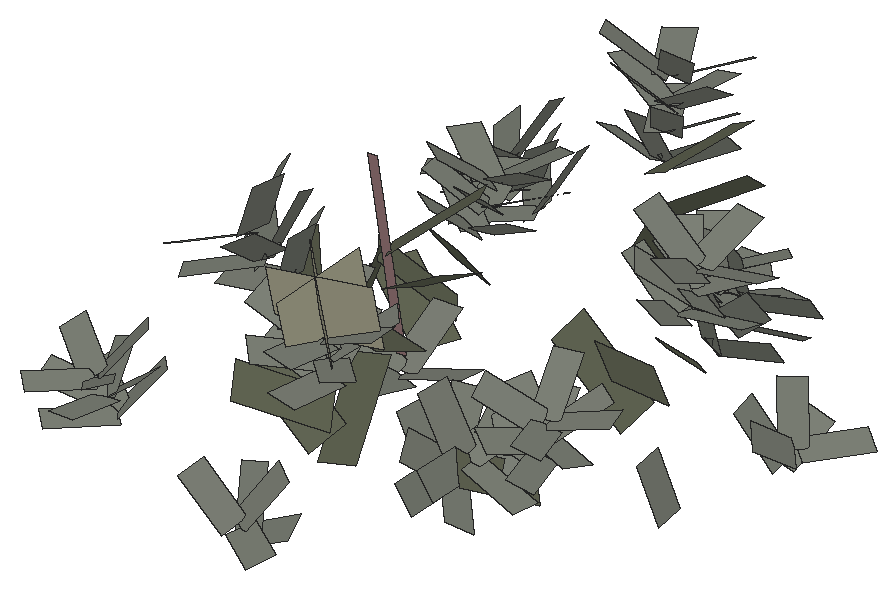
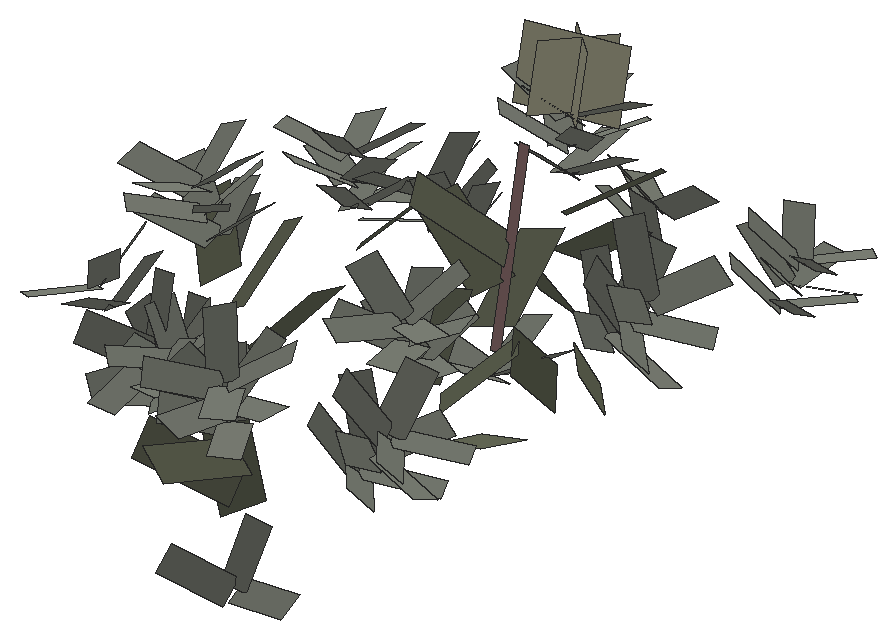
# SketchUp Ruby script. Lengths in inches.
U = 1.inch
M = Sketchup.active_model
def pt(a) = Geom::Point3d.new(a.map { |v| v * U })
def face(e, loops, mat)
  f = e.add_face(loops[0].map { |a| pt(a) })
  loops[1..].each { |l| e.add_face(l.map { |a| pt(a) }).erase! }
  f.material = f.back_material = mat if mat
  f
end
# faces: each face lists its corners as indices into pts; further lists are holes
def faces(e, pts, list, mat = nil) = list.each { |f| face(e, (f[0].is_a?(Array) ? f : [f]).map { |l| l.map { |i| pts[i] } }, mat) }
# xy, xz, yz: faces in a plane at the given z, y or x. An outline is a flat list of corners, or four numbers for a rectangle; further outlines are holes
def ring(l) = l.size == 4 ? [[l[0], l[1]], [l[2], l[1]], [l[2], l[3]], [l[0], l[3]]] : l.each_slice(2).to_a
def flat(e, list, mat, &to3) = list.each { |f| face(e, (f[0].is_a?(Array) ? f : [f]).map { |l| ring(l).map { |u, v| to3.(u, v) } }, mat) }
def xy(e, z, list, mat = nil) = flat(e, list, mat) { |x, y| [x, y, z] }
def xz(e, y, list, mat = nil) = flat(e, list, mat) { |x, z| [x, y, z] }
def yz(e, x, list, mat = nil) = flat(e, list, mat) { |y, z| [x, y, z] }
def lines(e, pts, list) = list.each { |a, b| e.add_line(pt(pts[a]), pt(pts[b])) }
# prism: a flat outline (further loops are holes) pulled along v
def prism(e, loops, v, mat = nil)
  f = face(e, loops, mat); d = Geom::Vector3d.new(v.map { |x| x * U })
  f.pushpull(f.normal.samedirection?(d) ? d.length : -d.length)
end
def box(e, o, s, mat = nil) = prism(e, [[o, [o[0] + s[0], o[1], o[2]], [o[0] + s[0], o[1] + s[1], o[2]], [o[0], o[1] + s[1], o[2]]]], [0, 0, s[2]], mat)
def at(x, y, z, deg = 0) = Geom::Transformation.translation(pt([x, y, z])) * Geom::Transformation.rotation(ORIGIN, Z_AXIS, deg.degrees)
def axes(o, x, y, z) = Geom::Transformation.new([*x, 0, *y, 0, *z, 0, *pt(o).to_a, 1])
def part(name) = M.definitions.add(name)
# library, detail: a bought-in or finely detailed component or shape, given as its bounding box
def library(name, o, s) = part(name).tap { |d| box(d.entities, o, s) }
def detail(e, o, s) = box(e.add_group.entities, o, s)
def put(e, d, t, mat = nil) = e.add_instance(d, t).tap { |i| i.material = mat if mat }
def group(e, t, mat = nil) = e.add_group.tap { |g| g.transformation = t; g.material = mat if mat }.entities
root = M.entities
M.materials.add("tak1dsfasd0f156w").color = [150, 118, 119]
M.materials.add("viburnumblaasdfas0df1w06d").color = [98, 102, 84]
M.materials.add("viburnumbladsadfasdfad0w122").color = [125, 129, 119]
M.materials.add("viburnumbloem2asdfas01vxc5016").color = [175, 173, 148]
c1 = part("Component\#315")
p = [[0.25,0,0],[2.05,0.01,0.35],[1.81,4.2,1.66],[0,4.19,1.3125]]
faces(c1.entities,p,[[0,1,2,3]],"viburnumbladsadfasdfad0w122")
c2 = part("viburnumblad2")
put(c2.entities,c1,axes([-19.23,-4.49,-32.18],[83.35428,0,0],[0,79.38502,0],[0,0,83.35428]))
c3 = part("Component\#314")
p = [[0.14,0,0],[2.58,0.05,0.25],[2.44,5.11,2.64],[0,5.05,2.39]]
faces(c3.entities,p,[[0,1,2,3]],"viburnumblaasdfas0df1w06d")
c4 = part("viburnumblad1\#2")
put(c4.entities,c3,axes([-37.25,6.23,19.31],[75.98784,0,0],[0,65.50676,0],[0,0,75.98784]))
c5 = part("Component\#336")
p = [[6.03,1.45,4.43],[5.85,2.68,0.17],[0,1.22,0],[0.18,0,4.25]]
faces(c5.entities,p,[[0,1,2,3]],"viburnumbloem2asdfas01vxc5016")
c6 = part("Component\#334")
p = [[0.16,3.84,5.17],[0,4.97,1.27],[3.78,1.125,0],[3.9375,0,3.9]]
faces(c6.entities,p,[[0,1,2,3]],"viburnumbloem2asdfas01vxc5016")
c7 = part("Component\#335")
p = [[1.35,5.21,5.35],[1.19,6.33,1.45],[0,1.125,0],[0.16,0,3.9]]
faces(c7.entities,p,[[0,1,2,3]],"viburnumbloem2asdfas01vxc5016")
c8 = part("Component\#337")
p = [[0.6,0,12.07],[1.51,1.22,0.03],[0.91,1.23,0],[0,0,12.04]]
faces(c8.entities,p,[[0,1,2,3]],"tak1dsfasd0f156w")
put(root,c2,axes([2210.91,323.67,41.88],[-0.00636,-0.00796,-0.00575],[0.0099,-0.00571,-0.00294],[-0.00097,-0.00646,0.0087]))
put(root,c2,axes([2209.49,322.42,40.99],[0.00636,0.00796,0.00575],[-0.00984,0.00398,0.00495],[0.00146,-0.00765,0.00773]))
put(root,c2,axes([2209.42,323.6,41.875],[0.00995,-0.00489,-0.00397],[0.00634,0.00703,0.00672],[-0.00053,-0.00802,0.00751]))
put(root,c2,axes([2209.95,324.8,40.99],[0.00254,-0.00908,-0.00688],[0.01053,0.00118,0.00207],[-0.00116,-0.00732,0.00806]))
put(root,c2,axes([2209.29,323.8125,40.29],[0.01153,0.00217,0.00126],[-0.00261,0.00855,0.00823],[0.00055,-0.00816,0.00738]))
put(root,c2,axes([2197.875,326.19,44.43],[-0.00773,0.00806,0.00054],[-0.00787,-0.00734,-0.00302],[-0.00183,-0.00247,0.01075]))
put(root,c2,axes([2198.58,327.34,43.45],[-0.01083,0.00076,-0.00267],[-0.00024,-0.01097,-0.00215],[-0.00276,-0.00202,0.01064]))
put(root,c2,axes([2198.09,327.5,44.91],[-0.00759,-0.00699,-0.00431],[0.00733,-0.00841,0.00072],[-0.00369,-0.00233,0.01029]))
put(root,c2,axes([2198.58,327.35,41.96],[-0.00742,0.00774,0.00052],[-0.0085,-0.00793,-0.00326],[-0.00183,-0.00247,0.01075]))
put(root,c2,axes([2197.65,326.64,42.95],[-0.0001,0.01064,0.00343],[-0.01164,0.00037,-0.00146],[-0.00143,-0.00341,0.01055]))
put(root,c2,axes([2197.74,328.5,43.6],[0.0001,-0.01064,-0.00343],[0.01052,-0.00118,0.00394],[-0.00407,-0.00322,0.0099]))
put(root,c2,axes([2211.68,329.93,50.16],[-0.01255,0.00027,0.0006],[-0.00036,-0.0124,-0.00196],[0.00055,-0.00198,0.01239]))
put(root,c2,axes([2196.52,326.51,44.17],[0.00759,0.00699,0.00431],[-0.00801,0.0076,0.00179],[-0.00181,-0.0043,0.01016]))
put(root,c2,axes([2196.74,327.82,44.66],[0.00773,-0.00806,-0.00054],[0.0072,0.00653,0.00553],[-0.00368,-0.00417,0.0097]))
put(root,c2,axes([2196.68,327.52,42.96],[0.01083,-0.00076,0.00267],[-0.0004,0.00932,0.00428],[-0.00274,-0.00461,0.00981]))
put(root,c2,axes([2211.3,331.08,47.23],[-0.01204,0.00026,0.00058],[-0.00039,-0.0134,-0.00212],[0.00055,-0.00198,0.01239]))
put(root,c2,axes([2211.14,329.92,48.49],[-0.00857,0.00873,0.00287],[-0.00949,-0.00914,-0.00056],[0.00162,-0.00243,0.01222]))
put(root,c2,axes([2197.19,327.55,41.69],[0.00793,0.00729,0.0045],[-0.00721,0.00684,0.00161],[-0.00181,-0.0043,0.01016]))
put(root,c2,axes([2197.3,328.65,42.17],[0.00743,-0.00696,-0.00145],[0.0072,0.00653,0.00553],[-0.00282,-0.00502,0.00959]))
put(root,c2,axes([2211.3125,331.27,48.9],[-0.00917,-0.00834,-0.00202],[0.00857,-0.00908,-0.00138],[-0.00054,-0.00239,0.01232]))
put(root,c4,axes([2210.54,330.9375,43.96],[-0.00623,0.01061,0.0062],[-0.01365,-0.00831,0.0005],[0.00356,-0.0051,0.0123]))
put(root,c5,axes([2207.86,328.26,49.92],[1.0472,0,0],[0,1.0472,0],[0,0,1.0472]))
put(root,c6,axes([2208.61,327.11,49.61],[1.0472,0,0],[0,1.0472,0],[0,0,1.0472]))
put(root,c2,axes([2210.35,329.08,49.97],[0.00042,0.01207,0.00346],[-0.01239,-0.00016,0.00207],[0.00203,-0.00348,0.0119]))
put(root,c7,axes([2210.11,326.48,49.53],[1.0472,0,0],[0,1.0472,0],[0,0,1.0472]))
put(root,c2,axes([2210.81,331.2,50.5625],[-0.00042,-0.01207,-0.00346],[0.01251,-0.00069,0.00087],[-0.00103,-0.00342,0.01205]))
put(root,c2,axes([2218.88,332.8125,43.26],[-0.00894,0.00051,0.00882],[-0.00128,-0.01248,-0.00058],[0.00874,-0.00131,0.00893]))
put(root,c2,axes([2210.04,330.1,47.05],[0.00044,0.0126,0.00361],[-0.01115,-0.00014,0.00186],[0.00203,-0.00348,0.0119]))
put(root,c2,axes([2209.66,329.84,48.52],[0.00917,0.00834,0.00202],[-0.00775,0.00756,0.00397],[0.00155,-0.00451,0.01162]))
put(root,c2,axes([2216.625,333.33,41.18],[-0.00933,0.00053,0.0092],[-0.00115,-0.01124,-0.00052],[0.00874,-0.00131,0.00893]))
put(root,c2,axes([2217.64,334.01,42.53],[-0.00797,-0.00829,0.00506],[0.00596,-0.00975,-0.0066],[0.00788,-0.0017,0.00963]))
put(root,c2,axes([2217.44,332.58,42.25],[-0.00467,0.00901,0.00741],[-0.00631,-0.00787,0.00559],[0.00942,-0.00179,0.00811]))
put(root,c4,axes([2209.14,331.31,41.85],[0.00552,0.01118,0.00587],[-0.01458,0.00491,0.00435],[0.00124,-0.00686,0.01189]))
put(root,c2,axes([2209.48,330.35,50.375],[0.01255,-0.00027,-0.0006],[0.00048,0.01156,0.0049],[0.00045,-0.00492,0.01155]))
put(root,c2,axes([2209.73,331.53,49.04],[0.00857,-0.00873,-0.00287],[0.00926,0.00794,0.00351],[-0.00062,-0.00447,0.01173]))
put(root,c2,axes([2217.79,331.97,44.05],[0.00233,0.01223,0.00166],[-0.00783,0.00016,0.00982],[0.00954,-0.00286,0.00766]))
put(root,c2,axes([2209.25,331.12,47.47],[0.01143,0.00024,-0.0017],[0.00048,0.01156,0.0049],[0.0018,-0.00492,0.01142]))
put(root,c2,axes([2218.47,334.11,44.07],[-0.00233,-0.01223,-0.00166],[0.00991,-0.00085,-0.00768],[0.00736,-0.00274,0.0098]))
put(root,c2,axes([2215.78,332.54,41.89],[0.00119,0.01147,0.00076],[-0.00783,0.00016,0.00982],[0.00974,-0.00152,0.00779]))
put(root,c2,axes([2222.57,335.72,46.21],[-0.01096,-0.00354,0.00194],[0.00316,-0.01102,-0.00224],[0.00251,-0.00157,0.0113]))
put(root,c2,axes([2221.92,335.55,44.73],[-0.00975,0.0051,0.00392],[-0.00563,-0.0109,0.00018],[0.00356,-0.00165,0.01101]))
put(root,c4,axes([2220.57,336.27,40.65],[-0.00789,0.00746,0.00681],[-0.00938,-0.01142,0.00165],[0.00606,-0.00342,0.01077]))
put(root,c2,axes([2221.56,336.62,43.59],[-0.01053,-0.0034,0.00186],[0.00341,-0.01191,-0.00242],[0.00251,-0.00157,0.0113]))
put(root,c2,axes([2216.2,332.64,43.52],[0.00797,0.00829,-0.00506],[-0.00363,0.00868,0.00851],[0.00902,-0.0039,0.00783]))
put(root,c2,axes([2221.65,334.58,46.15],[-0.00283,0.01075,0.0036],[-0.01053,-0.00387,0.00326],[0.00419,-0.00245,0.01063]))
put(root,c2,axes([2216.68,334.18,43.5625],[0.00467,-0.00901,-0.00741],[0.00895,0.00789,-0.00395],[0.00748,-0.00381,0.00935]))
put(root,c2,axes([2217.38,333.27,44.86],[0.00894,-0.00051,-0.00882],[0.00335,0.0118,0.00272],[0.00817,-0.00429,0.00853]))
put(root,c2,axes([2221.71,336.79,45.14],[-0.00575,-0.0101,-0.00117],[0.01003,-0.00542,-0.00255],[0.00167,-0.00226,0.01134]))
put(root,c4,axes([2208.125,333.28,39.75],[0.0147,-0.00029,0.00242],[-0.00086,0.01575,0.00709],[-0.00232,-0.00615,0.01338]))
put(root,c2,axes([2220.74,335.38,43.52],[-0.00295,0.01122,0.00376],[-0.00948,-0.00348,0.00294],[0.00419,-0.00245,0.01063]))
put(root,c2,axes([2221.48,336.58,46.72],[0.00283,-0.01075,-0.0036],[0.01123,0.00316,-0.00059],[0.00152,-0.00332,0.0111]))
put(root,c2,axes([2220.65,335.04,44.91],[0.00575,0.0101,0.00117],[-0.00857,0.00432,0.00479],[0.00404,-0.00351,0.01039]))
put(root,c2,axes([2220.56,335.43,46.66],[0.01096,0.00354,-0.00194],[-0.00246,0.01032,0.00491],[0.0032,-0.00419,0.01042]))
put(root,c2,axes([2220.27,336.55,45.45],[0.00975,-0.0051,-0.00392],[0.00612,0.00977,0.00252],[0.00215,-0.00412,0.01072]))
put(root,c2,axes([2219.79,336.04,44.04],[0.00971,0.00365,-0.00281],[-0.00246,0.01032,0.00491],[0.00437,-0.00379,0.01015]))
put(root,c2,axes([2198.02,339.73,48.33],[-0.00996,0.00362,-0.00815],[-0.00316,-0.01285,-0.00186],[-0.00834,0.00054,0.01043]))
put(root,c2,axes([2199.18,340.9375,47.21],[-0.00854,-0.00651,-0.00796],[0.00449,-0.01178,0.00482],[-0.00927,0.0004,0.00962]))
put(root,c4,axes([2207.59,342.11,42.92],[-0.0155,-0.00126,0.00308],[0.00163,-0.01831,0.00072],[0.00301,0.00088,0.01554]))
put(root,c2,axes([2198.72,339.38,46.66],[-0.00554,0.01163,-0.00356],[-0.00953,-0.00658,-0.00667],[-0.00756,-0.00023,0.01102]))
put(root,c2,axes([2226.6,339.36,39.98],[-0.00142,0.01147,0.00174],[-0.00575,-0.00222,0.00993],[0.01007,0.00035,0.00591]))
put(root,c2,axes([2197.51,341.32,48.06],[-0.00212,-0.01282,-0.00311],[0.00883,-0.00372,0.00932],[-0.00981,-0.00058,0.00906]))
put(root,c2,axes([2207.35,342.15,40.98],[-0.01323,-0.00019,0.0019],[0.00023,-0.01336,0.00026],[0.00189,0.00029,0.01323]))
put(root,c2,axes([2199.55,341.7,45.62],[-0.00096,-0.01167,-0.00375],[0.00883,-0.00372,0.00932],[-0.00998,-0.00196,0.00867]))
put(root,c2,axes([2199.27,339.62,44.98],[0.00203,0.01231,0.00299],[-0.01181,0.00375,-0.0074],[-0.00738,-0.00146,0.01104]))
put(root,c8,axes([2205.03,340.87,42.22],[1.0472,0,0],[0,1.0472,0],[0,0,1.0472]))
put(root,c2,axes([2197.8,341.45,46.03],[0.00554,-0.01163,0.00356],[0.00681,0.00581,0.00839],[-0.00964,-0.00181,0.00908]))
put(root,c4,axes([2206.57,343.19,45.8125],[-0.00531,-0.01357,0.00158],[0.01582,-0.00598,0.00178],[-0.00086,0.00203,0.01449]))
put(root,c2,axes([2205.98,341.16,41.08],[0,0.0133,0.00135],[-0.0129,-0.00035,0.00349],[0.0035,-0.0013,0.01283]))
put(root,c2,axes([2197.64,339.91,45.75],[0.00854,0.00651,0.00796],[-0.00689,0.01199,-0.00242],[-0.00792,-0.00244,0.01048]))
put(root,c2,axes([2196.33,340.76,46.99],[0.00996,-0.00362,0.00815],[0.00104,0.0126,0.00432],[-0.00886,-0.00258,0.00967]))
put(root,c2,axes([2206.38,343.51,41.26],[0,-0.0133,-0.00135],[0.01336,0.00003,-0.00028],[0.00028,-0.00135,0.01329]))
put(root,c2,axes([2198.63,341.16,44.64],[0.01039,-0.00378,0.00851],[0.00094,0.01134,0.00389],[-0.00886,-0.00258,0.00967]))
put(root,c4,axes([2200.69,340.79,41.91],[0.00849,0.00329,0.01149],[-0.00585,0.01597,-0.00025],[-0.01083,-0.00383,0.0091]))
put(root,c4,axes([2205.18,342.67,48.1],[0.00718,-0.01267,0.00168],[0.01433,0.00855,0.00326],[-0.00327,0.00004,0.01429]))
put(root,c4,axes([2202.2,342.375,40.29],[0.00719,-0.00894,0.00913],[0.00526,0.01343,0.009],[-0.01194,-0.00098,0.00844]))
put(root,c2,axes([2205.02,342.52,41.35],[0.01323,0.00019,-0.0019],[0.00023,0.01303,0.00294],[0.00189,-0.00295,0.0129]))
put(root,c4,axes([2220.42,347.33,41.85],[-0.01118,0.00552,0.00587],[-0.00491,-0.01458,0.00435],[0.00686,0.00124,0.01189]))
put(root,c4,axes([2220.79,348.73,43.96],[-0.01061,-0.00623,0.0062],[0.00831,-0.01365,0.0005],[0.0051,0.00356,0.0123]))
put(root,c2,axes([2221.63,348.23,47.05],[-0.0126,0.00044,0.00361],[0.00014,-0.01115,0.00186],[0.00348,0.00203,0.0119]))
put(root,c2,axes([2229.3125,347.68,40.99],[-0.00796,0.00636,0.00575],[-0.00398,-0.00984,0.00495],[0.00765,0.00146,0.00773]))
put(root,c2,axes([2222.65,348.54,49.97],[-0.01207,0.00042,0.00346],[0.00016,-0.01239,0.00207],[0.00348,0.00203,0.0119]))
put(root,c4,axes([2218.45,346.32,39.75],[0.00029,0.0147,0.00242],[-0.01575,-0.00086,0.00709],[0.00615,-0.00232,0.01338]))
put(root,c4,axes([2205.79,347.49,41.71],[-0.00837,0.01093,-0.00027],[-0.01213,-0.00903,0.00454],[0.00324,0.00308,0.01192]))
put(root,c2,axes([2221.89,347.85,48.52],[-0.00834,0.00917,0.00202],[-0.00756,-0.00775,0.00397],[0.00451,0.00155,0.01162]))
put(root,c2,axes([2221.82,349.33,48.49],[-0.00873,-0.00857,0.00287],[0.00914,-0.00949,-0.00056],[0.00243,0.00162,0.01222]))
put(root,c4,axes([2206.21,349.35,43.3],[-0.0135,0.00082,0.00242],[0.00046,-0.01443,0.00598],[0.00274,0.00585,0.01119]))
put(root,c2,axes([2227.92,347.48,40.29],[-0.00217,0.01153,0.00126],[-0.00855,-0.00261,0.00823],[0.00816,0.00055,0.00738]))
put(root,c2,axes([2220.61,347.44,47.47],[-0.00024,0.01143,-0.0017],[-0.01156,0.00048,0.0049],[0.00492,0.0018,0.01142]))
put(root,c2,axes([2221.39,347.67,50.375],[0.00027,0.01255,-0.0006],[-0.01156,0.00048,0.0049],[0.00492,0.00045,0.01155]))
put(root,c2,axes([2220.65,349.49,47.23],[-0.00026,-0.01204,0.00058],[0.0134,-0.00039,-0.00212],[0.00198,0.00055,0.01239]))
put(root,c4,axes([2204.2,346.54,39.48],[0.00652,0.01335,-0.00071],[-0.01553,0.00758,0.00028],[0.00058,0.00086,0.01356]))
put(root,c2,axes([2205.86,349.78,46.21],[-0.01136,0.00626,-0.00167],[-0.00561,-0.00886,0.00368],[0.00077,0.00497,0.01057]))
put(root,c2,axes([2221.8,349.87,50.16],[-0.00027,-0.01255,0.0006],[0.0124,-0.00036,-0.00196],[0.00198,0.00055,0.01239]))
put(root,c2,axes([2228.14,347.61,41.875],[0.00489,0.00995,-0.00397],[-0.00703,0.00634,0.00672],[0.00802,-0.00053,0.00751]))
put(root,c2,axes([2206.16,351.2,47.25],[-0.01214,-0.0031,0.00083],[0.00339,-0.01158,0.00463],[-0.0004,0.00512,0.01053]))
put(root,c2,axes([2206.1,350.78,48.91],[-0.01088,0.00599,-0.0016],[-0.00623,-0.00984,0.00409],[0.00077,0.00497,0.01057]))
put(root,c2,axes([2205.58,351.27,45.78],[-0.00603,-0.00996,0.00266],[0.01166,-0.00593,0.00316],[-0.00133,0.00444,0.01071]))
put(root,c2,axes([2220.2,347.92,49.04],[0.00873,0.00857,-0.00287],[-0.00794,0.00926,0.00351],[0.00447,-0.00062,0.01173]))
put(root,c2,axes([2226.93,348.14,40.99],[0.00908,0.00254,-0.00688],[-0.00118,0.01053,0.00207],[0.00732,-0.00116,0.00806]))
put(root,c2,axes([2228.0625,349.1,41.88],[0.00796,-0.00636,-0.00575],[0.00571,0.0099,-0.00294],[0.00646,-0.00097,0.0087]))
put(root,c2,axes([2220.47,349.5,48.9],[0.00834,-0.00917,-0.00202],[0.00908,0.00857,-0.00138],[0.00239,-0.00054,0.01232]))
put(root,c2,axes([2205.52,349.92,47.58],[-0.00325,0.01157,-0.00309],[-0.01106,-0.00241,0.00198],[0.00148,0.00409,0.01081]))
put(root,c2,axes([2205.96,352.29,48.5],[-0.00628,-0.01038,0.00277],[0.0108,-0.00549,0.00293],[-0.00133,0.00444,0.01071]))
put(root,c2,axes([2220.53,349,50.5625],[0.01207,-0.00042,-0.00346],[0.00069,0.01251,0.00087],[0.00342,-0.00103,0.01205]))
put(root,c2,axes([2204.53,349.63,46.35],[0.00561,0.0092,-0.00364],[-0.0108,0.0064,-0.00025],[0.002,0.00408,0.01074]))
put(root,c2,axes([2205,351.98,47.07],[0.00325,-0.01157,0.00309],[0.01204,0.00353,0.00052],[-0.00148,0.00333,0.01101]))
put(root,c2,axes([2204.52,350.65,48.94],[0.00628,0.01038,-0.00277],[-0.0108,0.0064,-0.00025],[0.00133,0.00298,0.0111]))
put(root,c2,axes([2203.99,350.78,47.38],[0.01214,0.0031,-0.00083],[-0.00326,0.01206,-0.00174],[0.0004,0.0023,0.01128]))
put(root,c2,axes([2219.19,353.97,41.89],[-0.01147,0.00119,0.00076],[-0.00016,-0.00783,0.00982],[0.00152,0.00974,0.00779]))
put(root,c2,axes([2204.38,352.15,48.54],[0.01088,-0.00599,0.0016],[0.00623,0.01076,-0.00141],[-0.00077,0.00244,0.01124]))
put(root,c2,axes([2218.4,354.82,41.18],[-0.00053,-0.00933,0.0092],[0.01124,-0.00115,-0.00052],[0.00131,0.00874,0.00893]))
put(root,c2,axes([2219.16,355.63,42.25],[-0.00901,-0.00467,0.00741],[0.00787,-0.00631,0.00559],[0.00179,0.00942,0.00811]))
put(root,c2,axes([2219.09,354.4,43.52],[-0.00829,0.00797,-0.00506],[-0.00868,-0.00363,0.00851],[0.0039,0.00902,0.00783]))
put(root,c2,axes([2216.69,355.3125,42.43],[-0.00726,0.00696,-0.0015],[-0.00749,-0.00689,0.00431],[0.00194,0.00418,0.01005]))
put(root,c2,axes([2216.83,356.43,42.06],[-0.00812,-0.00757,0.00318],[0.00703,-0.00685,0.00164],[0.0009,0.00343,0.01047]))
put(root,c2,axes([2217.23,356.36,43.35],[-0.0109,0.00051,0.00178],[0.00012,-0.00953,0.00349],[0.00185,0.00377,0.01023]))
put(root,c2,axes([2219.76,355.98,44.05],[-0.01223,0.00233,0.00166],[-0.00016,-0.00783,0.00982],[0.00286,0.00954,0.00766]))
put(root,c2,axes([2217.03,355.93,44.98],[-0.00764,0.00797,-0.00053],[-0.00749,-0.00689,0.00431],[0.00278,0.00334,0.01017]))
put(root,c2,axes([2217.27,357.26,44.63],[-0.00778,-0.00725,0.00304],[0.00781,-0.00761,0.00182],[0.0009,0.00343,0.01047]))
put(root,c2,axes([2202.85,357.25,44.97],[-0.00962,0.00434,-0.00682],[-0.00417,-0.01174,-0.00159],[-0.00692,0.00104,0.01043]))
put(root,c2,axes([2201.98,357.89,46.33],[-0.00913,-0.00526,-0.00683],[0.00354,-0.01136,0.00402],[-0.00787,0.001,0.00974]))
put(root,c2,axes([2216.14,355.35,43.81],[0.0001,0.01076,-0.00253],[-0.0107,0.00082,0.00309],[0.00316,0.0024,0.01032]))
put(root,c2,axes([2201.36,356.52,45.83],[-0.00447,0.0114,-0.0028],[-0.00996,-0.00527,-0.00554],[-0.00621,0.00025,0.01092]))
put(root,c2,axes([2217.72,355.83,42.53],[0.00829,-0.00797,0.00506],[0.00975,0.00596,-0.0066],[0.0017,0.00788,0.00963]))
put(root,c2,axes([2216.26,357.24,43.33],[-0.0001,-0.01076,0.00253],[0.0116,-0.00022,-0.00049],[0.00051,0.00252,0.01075]))
put(root,c2,axes([2218.92,357.07,43.26],[-0.00051,-0.00894,0.00882],[0.01248,-0.00128,-0.00058],[0.00131,0.00874,0.00893]))
put(root,c2,axes([2203.32,356.97,43.38],[-0.00429,0.01094,-0.00269],[-0.01076,-0.0057,-0.00599],[-0.00621,0.00025,0.01092]))
put(root,c2,axes([2217.55,354.87,43.5625],[0.00901,0.00467,-0.00741],[-0.00789,0.00895,-0.00395],[0.00381,0.00748,0.00935]))
put(root,c2,axes([2218.46,355.57,44.86],[0.00051,0.00894,-0.00882],[-0.0118,0.00335,0.00272],[0.00429,0.00817,0.00853]))
put(root,c2,axes([2202.46,358.8,44.74],[-0.0033,-0.01178,-0.00285],[0.00874,-0.0044,0.00808],[-0.00849,0.00014,0.00926]))
put(root,c2,axes([2215.44,356.61,42.22],[0.00733,-0.00766,0.00051],[0.00858,0.00809,-0.00187],[0.00089,0.00157,0.01091]))
put(root,c2,axes([2215.67,356.23,45.15],[0.00778,0.00725,-0.00304],[-0.00736,0.00822,0.00077],[0.00276,0.00149,0.0106]))
put(root,c2,axes([2201.79,356.77,44.15],[0.0033,0.01178,0.00285],[-0.01097,0.00447,-0.0058],[-0.00615,-0.00092,0.01092]))
put(root,c2,axes([2215.32,356.5,43.6875],[0.0109,-0.00051,-0.00178],[0.00032,0.01098,-0.00121],[0.00182,0.00115,0.01084]))
put(root,c2,axes([2215.92,357.56,44.8],[0.00764,-0.00797,0.00053],[0.00794,0.00749,-0.00173],[0.00089,0.00157,0.01091]))
put(root,c2,axes([2217.62,356.66,44.07],[0.01223,-0.00233,-0.00166],[0.00085,0.00991,-0.00768],[0.00274,0.00736,0.0098]))
put(root,c2,axes([2200.85,358.68,45.54],[0.00447,-0.0114,0.0028],[0.00817,0.00518,0.00802],[-0.00843,-0.00103,0.00925]))
put(root,c2,axes([2202.53,358.85,43.05],[0.00493,-0.01032,0.00165],[0.00817,0.00518,0.00802],[-0.0079,-0.00226,0.0095]))
put(root,c2,axes([2200.24,357.3125,45.04],[0.00913,0.00526,0.00683],[-0.00534,0.01127,-0.00154],[-0.00678,-0.00178,0.01043]))
put(root,c2,axes([2201.19,358.0625,43.74],[0.00962,-0.00434,0.00682],[0.00218,0.01069,0.00373],[-0.00772,-0.00183,0.00974]))
put(root,c2,axes([2202.11,357.65,42.58],[0.00954,0.0055,0.00713],[-0.0048,0.01014,-0.00139],[-0.00678,-0.00178,0.01043]))
put(root,c4,axes([2209.09,361.62,39.45],[-0.01228,-0.00656,0.00533],[0.00976,-0.01204,0.00766],[0.00081,0.00845,0.01225]))
put(root,c2,axes([2208.17,364.11,47.11],[-0.00983,-0.00604,0.00067],[0.00618,-0.00942,0.00556],[-0.00236,0.00509,0.01124]))
put(root,c2,axes([2208.2,363.75,48.76],[-0.01213,0.00288,-0.00157],[-0.00331,-0.01081,0.00577],[-0.00003,0.00592,0.01108]))
put(root,c2,axes([2208.01,365.1,49.94],[-0.01088,-0.00598,0.00194],[0.00618,-0.00942,0.00556],[-0.00119,0.00576,0.0111]))
put(root,c2,axes([2207.34,363.75,50.45],[-0.00627,0.01006,-0.00416],[-0.01085,-0.00538,0.00335],[0.0009,0.00527,0.01137]))
put(root,c4,axes([2207.54,363.14,41.6],[0.00185,-0.01141,0.00751],[0.01551,0.00355,0.00158],[-0.0028,0.0071,0.01148]))
put(root,c2,axes([2207.32,365.16,48.14],[-0.00325,-0.01134,0.00432],[0.011,-0.00211,0.00274],[-0.0019,0.00489,0.01141]))
put(root,c2,axes([2206.7,363.19,48.93],[0.00325,0.01134,-0.00432],[-0.01209,0.00342,-0.00014],[0.00105,0.00419,0.0118]))
put(root,c2,axes([2206.92,364.53,46.79],[0.00655,-0.0105,0.00435],[0.00967,0.00585,-0.00045],[-0.00175,0.00381,0.01184]))
put(root,c2,axes([2206.38,363.1,47.28],[0.01044,0.00574,-0.00186],[-0.00678,0.01138,-0.00292],[0.00034,0.00331,0.01211]))
put(root,c4,axes([2206.47,363.1,43.93],[0.01159,-0.00514,0.00541],[0.00744,0.01388,-0.00276],[-0.00381,0.00452,0.01245]))
put(root,c2,axes([2206.57,365.7,49.65],[0.00627,-0.01006,0.00416],[0.01074,0.0065,-0.0005],[-0.00175,0.00381,0.01184]))
put(root,c2,axes([2206.1,364.37,48.42],[0.01213,-0.00288,0.00157],[0.00334,0.0124,-0.003],[-0.00082,0.00316,0.01213]))
put(root,c2,axes([2205.9,364.35,50.16],[0.01088,0.00598,-0.00194],[-0.00628,0.01054,-0.00271],[0.00034,0.00331,0.01211]))
put(root,c2,axes([2203.39,369.64,41.24],[-0.01151,-0.00126,-0.00215],[-0.00083,-0.00812,0.00826],[-0.00252,0.0083,0.00677]))
put(root,c2,axes([2202.16,368.85,41.55],[0.00052,0.00907,-0.00737],[-0.01174,-0.00037,-0.00119],[-0.00118,0.00734,0.00793]))
put(root,c2,axes([2202.6,370.48,40.32],[-0.00052,-0.00907,0.00737],[0.0111,0.00213,0.00308],[-0.00399,0.00704,0.00741]))
